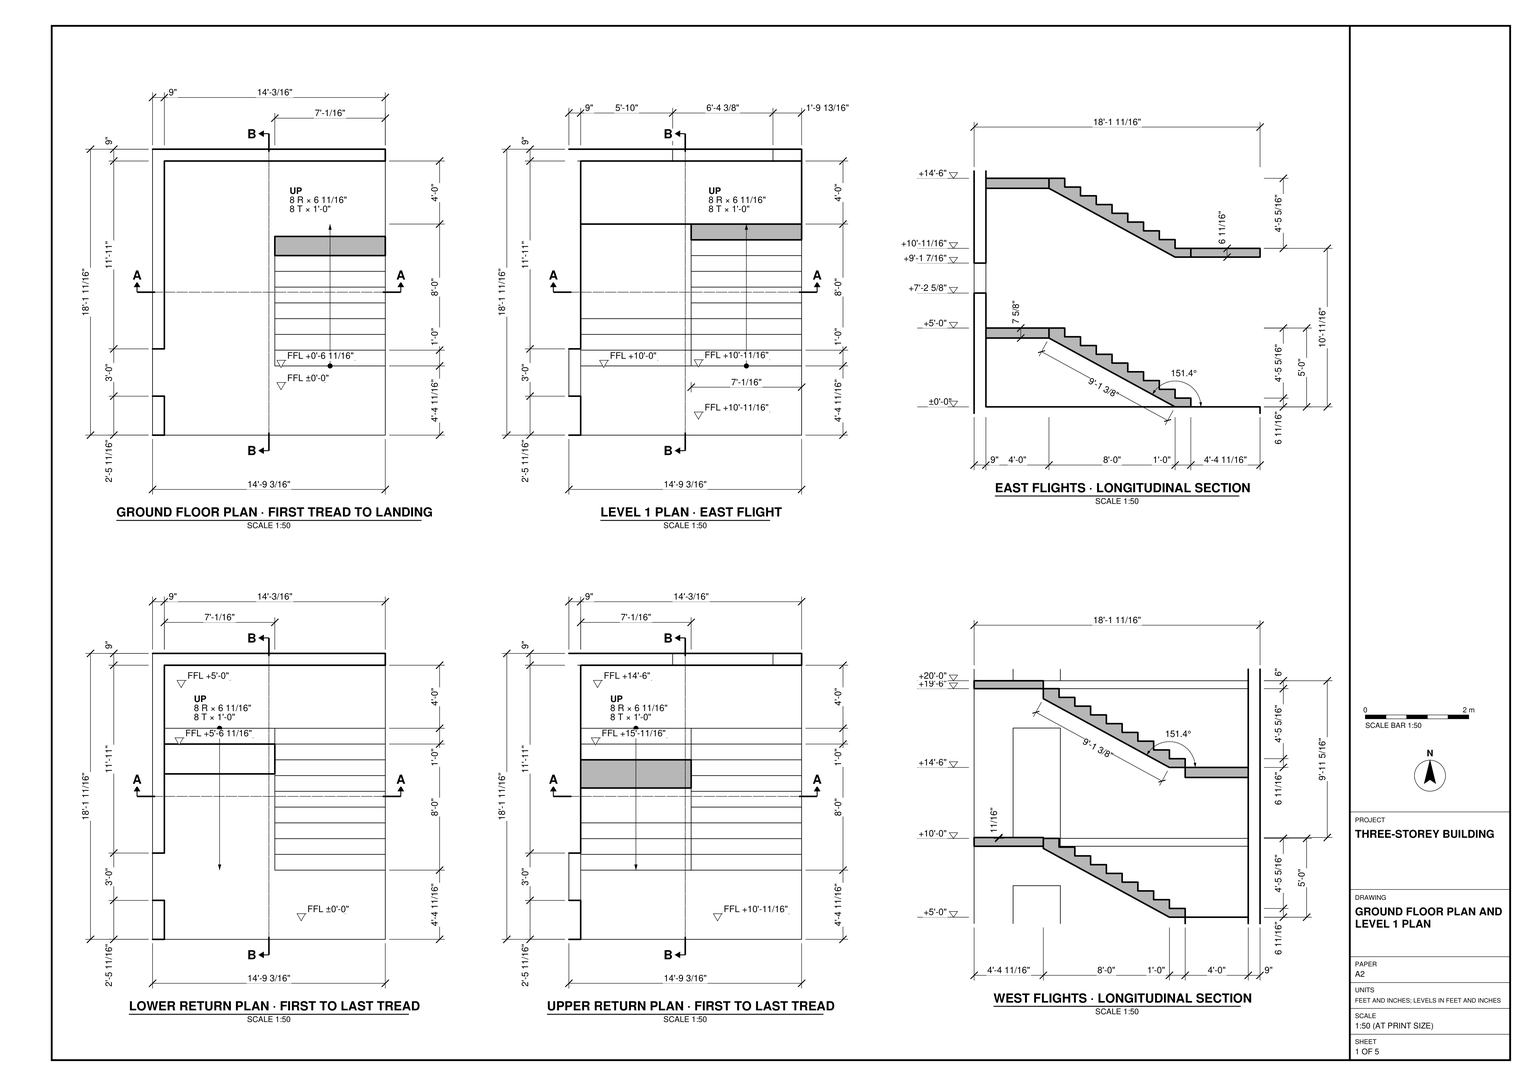
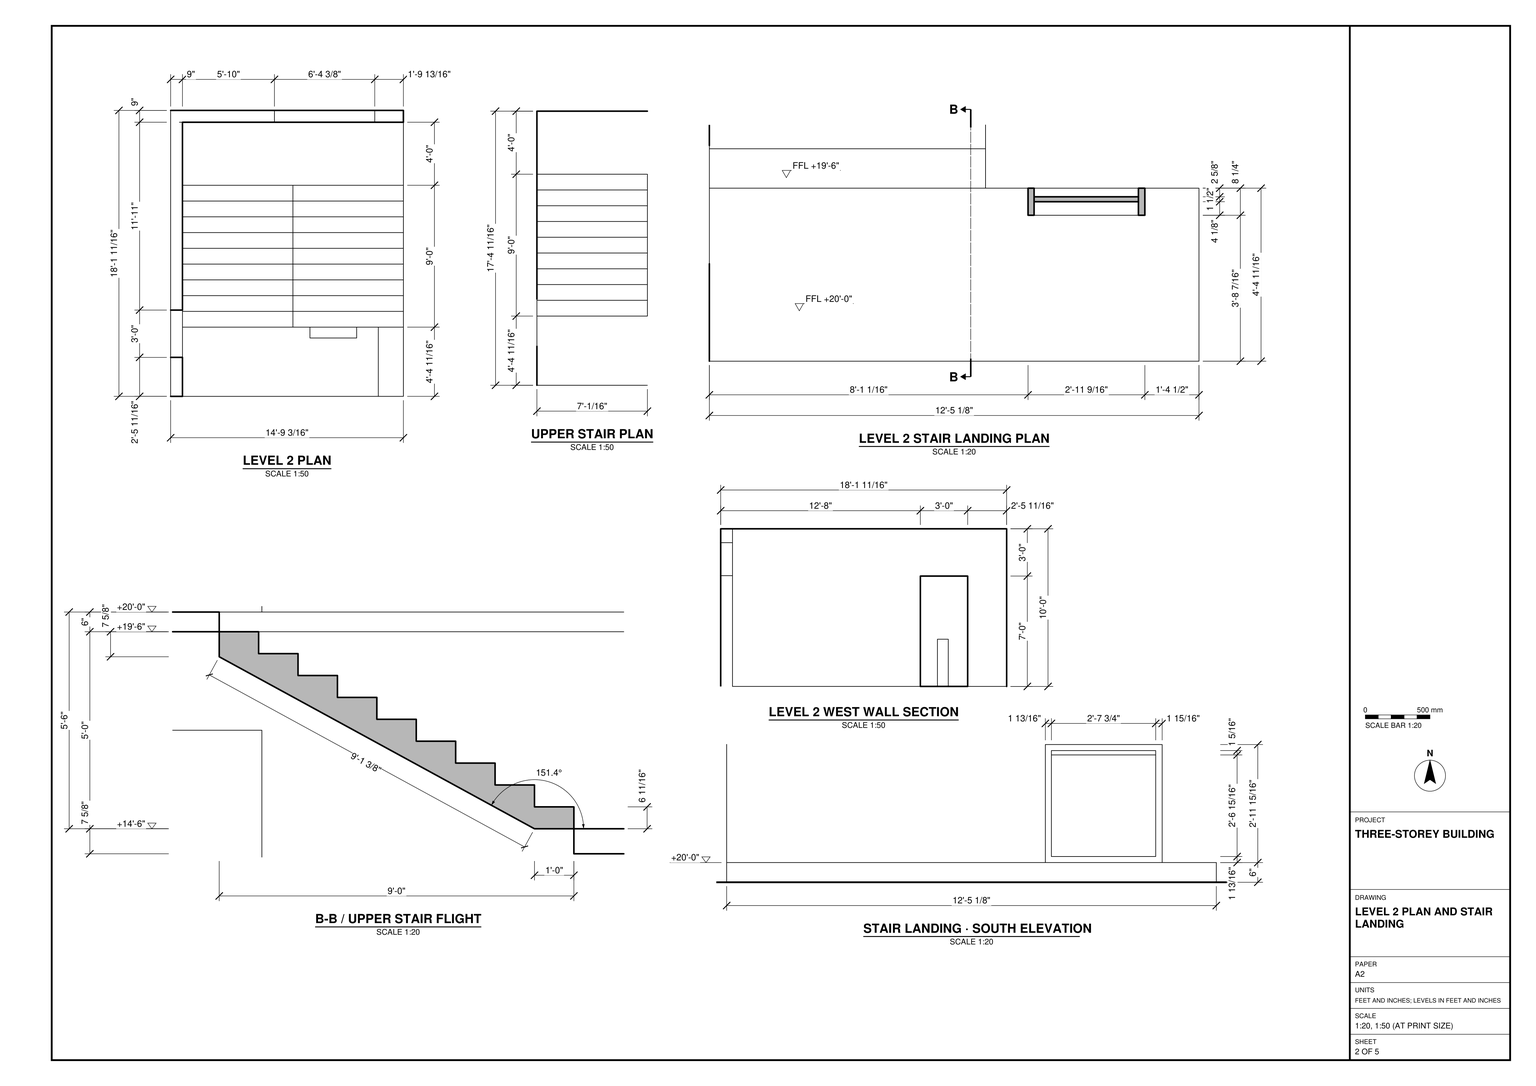
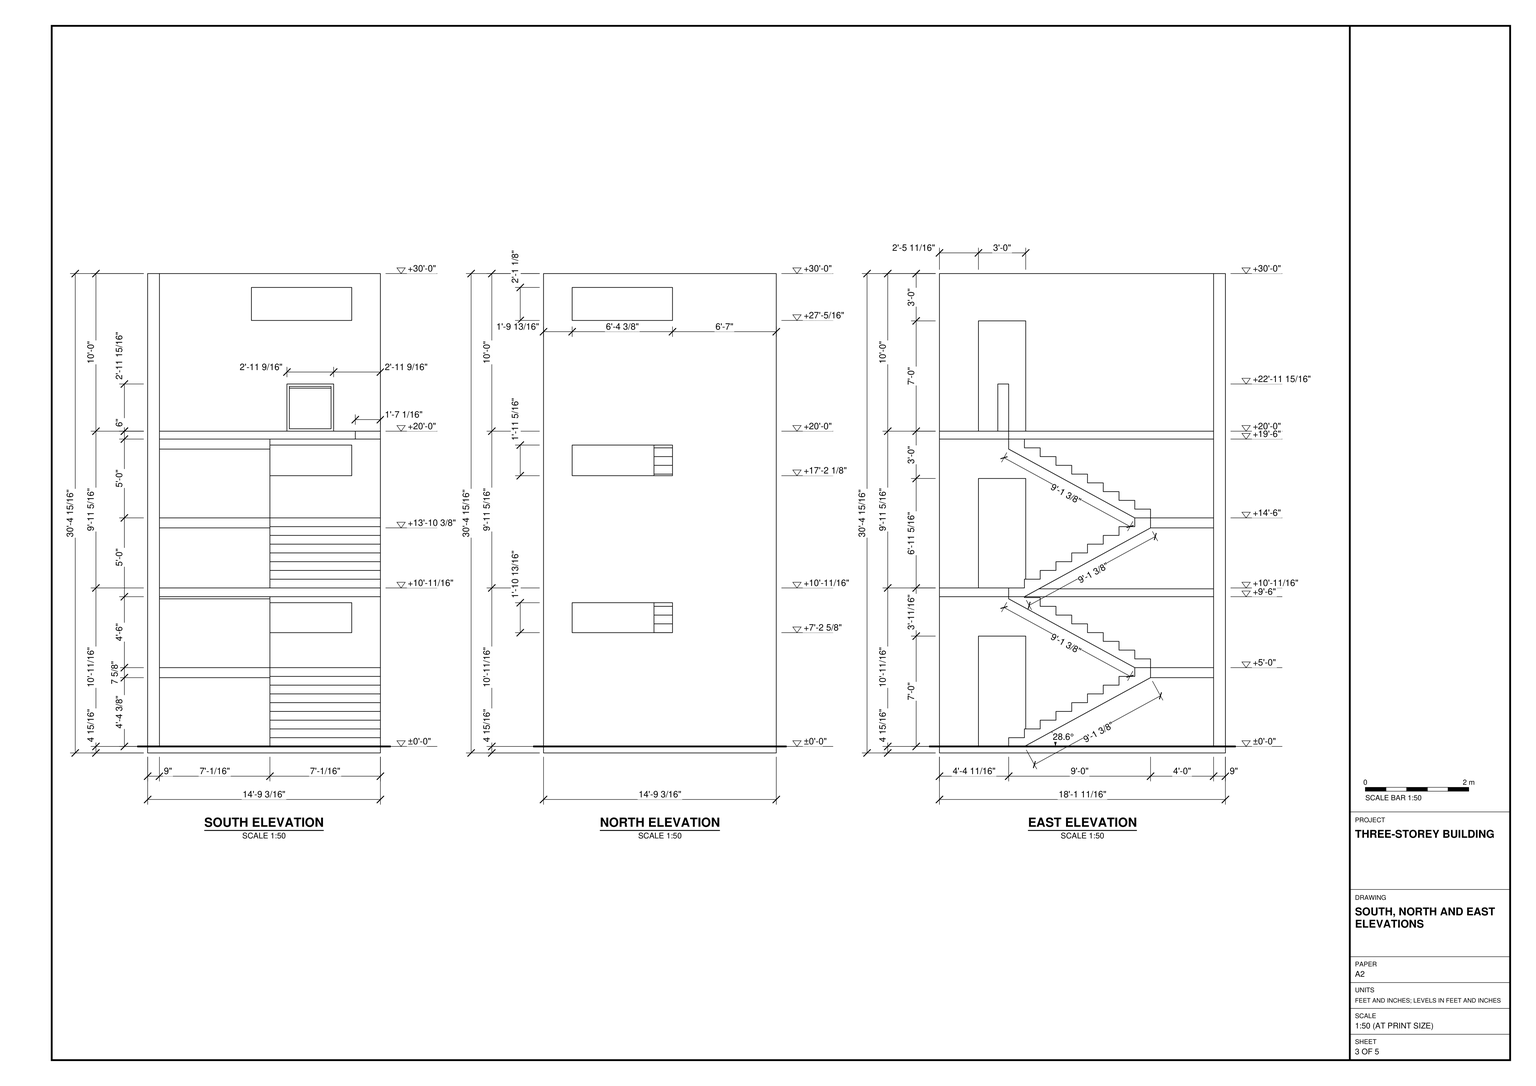
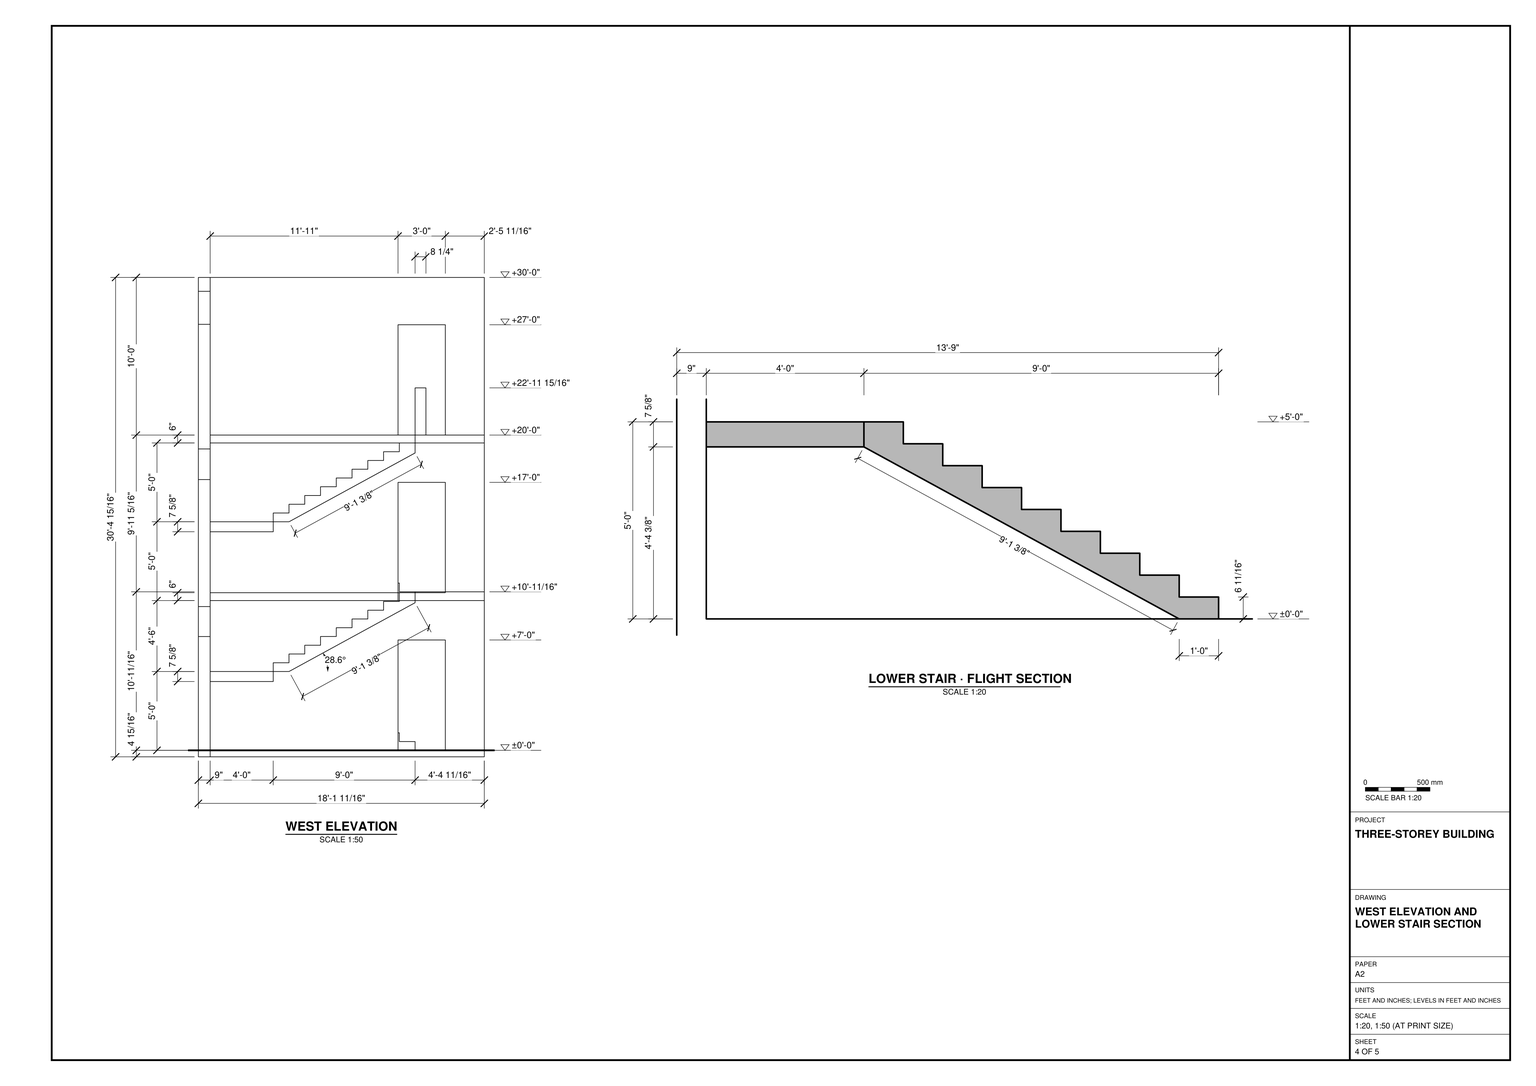
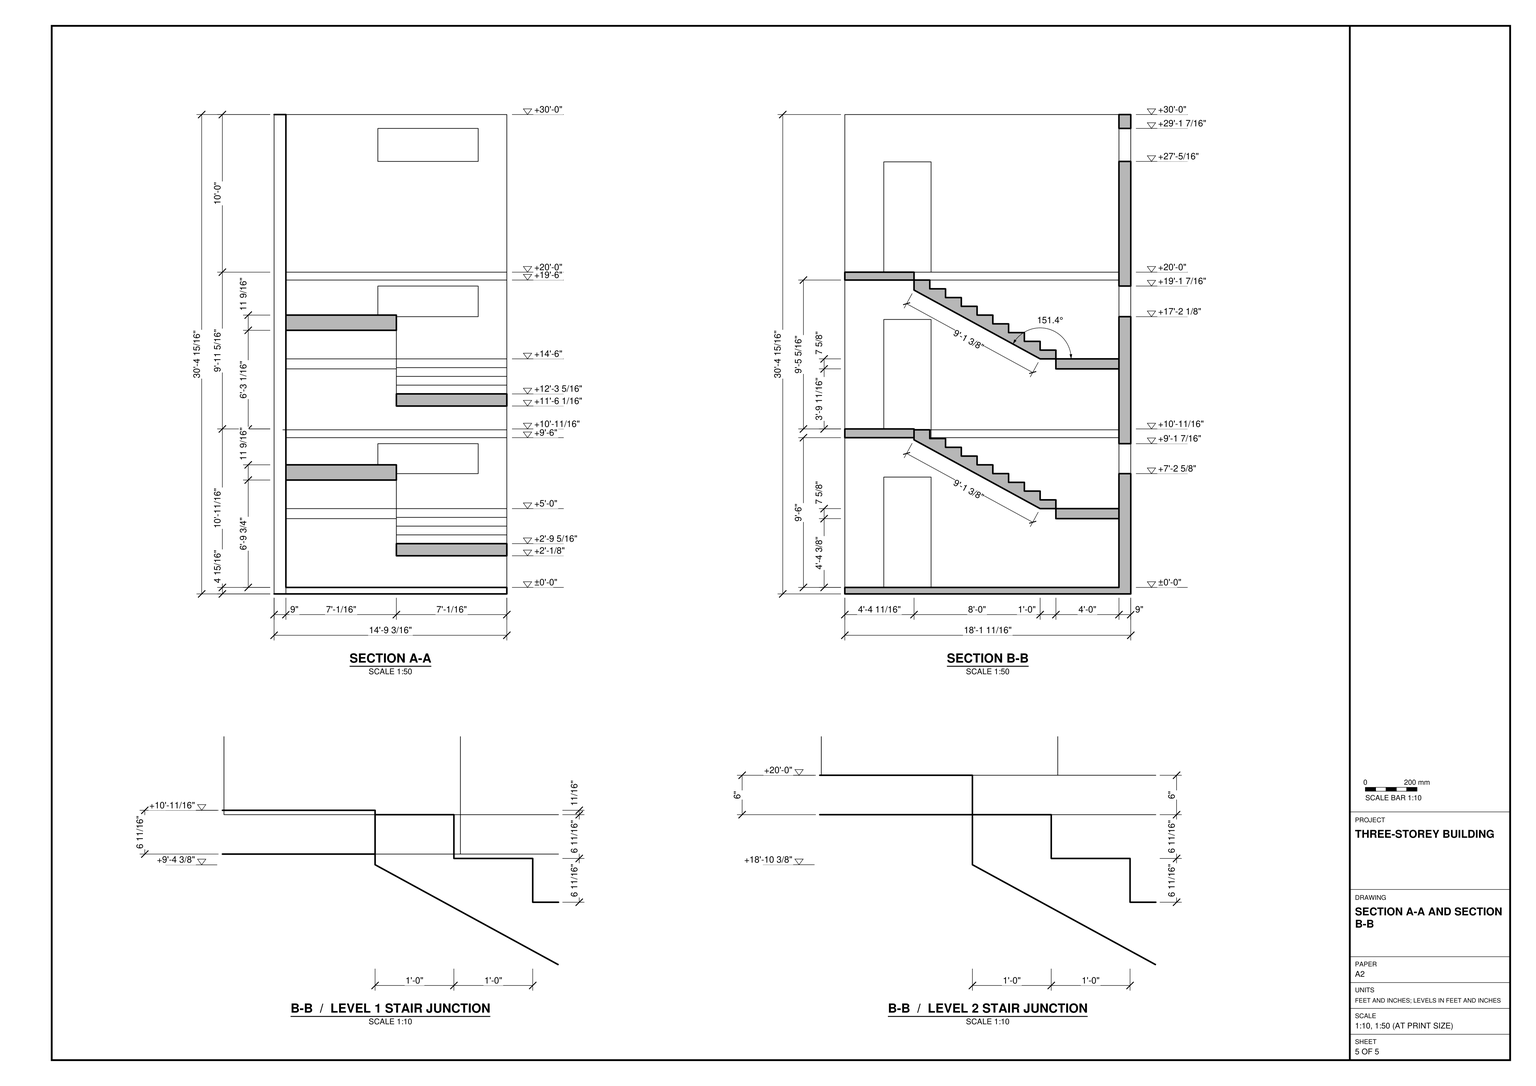
Build the stairwell shown in task_files/diagram_01.pdf in SketchUp. Work in feet and inches. Set the overall east–west width to 14'-9 3/16", the north–south depth to 18'-1 11/16", and the total height, including the base slab, to 30'-4 15/16". Use finished floor levels of ±0'-0", +10'-11/16", and +20'-0".

Form the north and west walls at the drawn 9" thickness. Cut the horizontal window openings in the north wall and the door openings near the south end of the west wall. Leave the flights visible from the open sides as shown in the elevations.

Start the stair on the east side, ascend toward the north landing, then turn back along the west side to reach the next floor. Repeat this arrangement up to the top floor. Model the individual treads and risers, sloping undersides, and flat landing slabs. Use the sections to distinguish each floor landing from its adjacent tread. Include the small element shown near the east end of the top floor landing.

Keep the walls, slabs, stair flights, and each furniture or joinery piece separate as groups or components, and use components for repeated parts. Any decor or loose items shown may be suitable library components. Save one SketchUp model as output_files/three_storey_switchback_stairwell.skp.

# SketchUp Ruby script. Lengths in inches.
U = 1.inch
M = Sketchup.active_model
def pt(a) = Geom::Point3d.new(a.map { |v| v * U })
def face(e, loops, mat)
  f = e.add_face(loops[0].map { |a| pt(a) })
  loops[1..].each { |l| e.add_face(l.map { |a| pt(a) }).erase! }
  f.material = f.back_material = mat if mat
  f
end
# faces: each face lists its corners as indices into pts; further lists are holes
def faces(e, pts, list, mat = nil) = list.each { |f| face(e, (f[0].is_a?(Array) ? f : [f]).map { |l| l.map { |i| pts[i] } }, mat) }
# xy, xz, yz: faces in a plane at the given z, y or x. An outline is a flat list of corners, or four numbers for a rectangle; further outlines are holes
def ring(l) = l.size == 4 ? [[l[0], l[1]], [l[2], l[1]], [l[2], l[3]], [l[0], l[3]]] : l.each_slice(2).to_a
def flat(e, list, mat, &to3) = list.each { |f| face(e, (f[0].is_a?(Array) ? f : [f]).map { |l| ring(l).map { |u, v| to3.(u, v) } }, mat) }
def xy(e, z, list, mat = nil) = flat(e, list, mat) { |x, y| [x, y, z] }
def xz(e, y, list, mat = nil) = flat(e, list, mat) { |x, z| [x, y, z] }
def yz(e, x, list, mat = nil) = flat(e, list, mat) { |y, z| [x, y, z] }
def lines(e, pts, list) = list.each { |a, b| e.add_line(pt(pts[a]), pt(pts[b])) }
# prism: a flat outline (further loops are holes) pulled along v
def prism(e, loops, v, mat = nil)
  f = face(e, loops, mat); d = Geom::Vector3d.new(v.map { |x| x * U })
  f.pushpull(f.normal.samedirection?(d) ? d.length : -d.length)
end
def box(e, o, s, mat = nil) = prism(e, [[o, [o[0] + s[0], o[1], o[2]], [o[0] + s[0], o[1] + s[1], o[2]], [o[0], o[1] + s[1], o[2]]]], [0, 0, s[2]], mat)
def at(x, y, z, deg = 0) = Geom::Transformation.translation(pt([x, y, z])) * Geom::Transformation.rotation(ORIGIN, Z_AXIS, deg.degrees)
def axes(o, x, y, z) = Geom::Transformation.new([*x, 0, *y, 0, *z, 0, *pt(o).to_a, 1])
def part(name) = M.definitions.add(name)
# library, detail: a bought-in or finely detailed component or shape, given as its bounding box
def library(name, o, s) = part(name).tap { |d| box(d.entities, o, s) }
def detail(e, o, s) = box(e.add_group.entities, o, s)
def put(e, d, t, mat = nil) = e.add_instance(d, t).tap { |i| i.material = mat if mat }
def group(e, t, mat = nil) = e.add_group.tap { |g| g.transformation = t; g.material = mat if mat }.entities
root = M.entities
M.materials.add("[Translucent Glass Gray]").color = [51, 51, 51]
M.materials["[Translucent Glass Gray]"].alpha = 0.5
c1 = part("Group\#1")
prism(c1.entities,[[[48,12,0],[48,108,55],[48,108,63],[48,96,63],[48,96,56],[48,84,56],[48,84,49],[48,72,49],[48,72,42],[48,60,42],[48,60,35],[48,48,35],[48,48,28],[48,36,28],[48,36,21],[48,24,21],[48,24,14],[48,12,14],[48,12,7],[48,0,7],[48,0,0],[48,8,0]]],[-48,0,0])
c2 = part("Group\#3")
g1 = group(c2.entities,at(96,108,55))
box(g1,[-96,0,0],[96,48,8])
put(c2.entities,c1,at(48,0,0))
put(c2.entities,c1,at(48,108,63,-180))
xy(root,-4.9375,[[0,0,177.1875,217.6875]])
xy(root,0,[[9,0,177.1875,0,177.1875,208.6875,9,208.6875,9,65.68,0,65.68,0,29.68,9,29.68]])
xy(root,84,[[0,29.68,9,65.68]])
xy(root,86.625,[[79.01,208.6875,155.38,217.6875]])
xy(root,109.4375,[[79.01,208.6875,155.38,217.6875]])
xy(root,114,[[9,0,177.1875,52.6875]])
xy(root,120,[[0,29.68,9,65.68]])
xy(root,120.67,[[9,0,177.1875,52.6875]])
xy(root,204,[[0,29.68,9,65.68]])
xy(root,206.125,[[79.01,208.6875,155.38,217.6875]])
xy(root,229.4375,[[79.01,208.6875,155.38,217.6875]])
xy(root,234,[[9,0,158.09,52.6875]])
xy(root,240,[[9,0,158.09,0,158.09,52.6875,141.61,52.6875,141.61,44.4375,106.04,44.4375,106.04,52.6875,9,52.6875],[0,29.68,9,65.68],[106.04,44.4375,112.47,52.6875],[112.47,44.4375,141.61,52.6875]])
xy(root,241.84,[[107.88,44.4375,139.65,48.5625],[107.88,48.5625,139.65,50.0625],[107.88,50.0625,139.65,52.6875]])
xy(root,272.78,[[107.88,48.5625,139.65,50.0625]])
xy(root,274.1,[[107.88,44.4375,139.65,52.6875]])
xy(root,275.9375,[[106.04,44.4375,141.61,52.6875]])
xy(root,324,[[0,29.68,9,65.68]])
xy(root,324.3125,[[79.01,208.6875,155.38,217.6875]])
xy(root,349.4375,[[79.01,208.6875,155.38,217.6875]])
xy(root,360,[[0,0,9,0,9,208.6875,177.1875,208.6875,177.1875,217.6875,0,217.6875]])
xz(root,0,[[0,-4.9375,177.1875,0],[0,0,9,360],[9,114,177.1875,120.67],[9,234,158.09,240]])
xz(root,29.68,[[0,0,9,84],[0,120,9,204],[0,240,9,324]])
xz(root,44.4375,[[[106.04,240,141.61,275.9375],[107.88,241.84,139.65,274.1]]])
xz(root,48.5625,[[107.88,241.84,139.65,272.78]],"[Translucent Glass Gray]")
xz(root,50.0625,[[107.88,241.84,139.65,272.78]],"[Translucent Glass Gray]")
xz(root,52.6875,[[9,114,177.1875,120.67],[9,234,158.09,240],[[106.04,240,141.61,275.9375],[107.88,241.84,139.65,274.1]]])
xz(root,65.68,[[0,0,9,84],[0,120,9,204],[0,240,9,324]])
xz(root,208.6875,[[[9,0,177.1875,114],[79.01,86.625,155.38,109.4375]],[9,114,177.1875,120],[[9,120,177.1875,234],[79.01,206.125,155.38,229.4375]],[9,234,177.1875,240],[[9,240,177.1875,360],[79.01,324.3125,155.38,349.4375]]])
xz(root,217.6875,[[[0,-4.9375,177.1875,360],[79.01,324.3125,155.38,349.4375],[79.01,206.125,155.38,229.4375],[79.01,86.625,155.38,109.4375]]])
yz(root,9,[[0,0,29.68,0,29.68,84,65.68,84,65.68,0,208.6875,0,208.6875,114,0,114],[0,114,0,120.67,29.68,120.67,29.68,120,52.6875,120,52.6875,114],[52.6875,114,65.68,120],[65.68,114,208.6875,120],[65.68,120,208.6875,120,208.6875,234,0,234,0,120.67,29.68,120.67,29.68,204,65.68,204],
  [29.68,120,52.6875,120.67],[0,234,52.6875,240],[52.6875,234,208.6875,240],[0,240,29.68,240,29.68,324,65.68,324,65.68,240,208.6875,240,208.6875,360,0,360]])
yz(root,79.01,[[208.6875,86.625,217.6875,109.4375],[208.6875,206.125,217.6875,229.4375],[208.6875,324.3125,217.6875,349.4375]])
yz(root,106.04,[[44.4375,240,52.6875,275.9375]])
yz(root,107.88,[[44.4375,241.84,48.5625,241.84,48.5625,272.78,50.0625,272.78,50.0625,241.84,52.6875,241.84,52.6875,274.1,44.4375,274.1],[48.5625,241.84,50.0625,272.78]])
yz(root,139.65,[[44.4375,241.84,44.4375,274.1,52.6875,274.1,52.6875,241.84,50.0625,241.84,50.0625,272.78,48.5625,272.78,48.5625,241.84],[48.5625,241.84,50.0625,272.78]])
yz(root,141.61,[[44.4375,240,52.6875,275.9375]])
yz(root,155.38,[[208.6875,86.625,217.6875,109.4375],[208.6875,206.125,217.6875,229.4375],[208.6875,324.3125,217.6875,349.4375]])
yz(root,158.09,[[0,234,52.6875,240]])
yz(root,177.1875,[[0,-4.9375,217.6875,-4.9375,217.6875,360,208.6875,360,208.6875,0,0,0],[0,114,52.6875,120.67]])
p = [[9,208.6875,-4.9375],[177.1875,208.6875,-4.9375],[9,208.6875,0],[9,208.6875,120],[6.64,208.6875,120]]
lines(root,p,[[0,1],[2,0],[3,4]])
put(root,c2,axes([9,52.6875,0],[1.75195,0,0],[0,1,0],[0,0,0.95238]))
put(root,c2,axes([9,52.6875,114],[1.75195,0,0],[0,1,0],[0,0,0.95238]))
